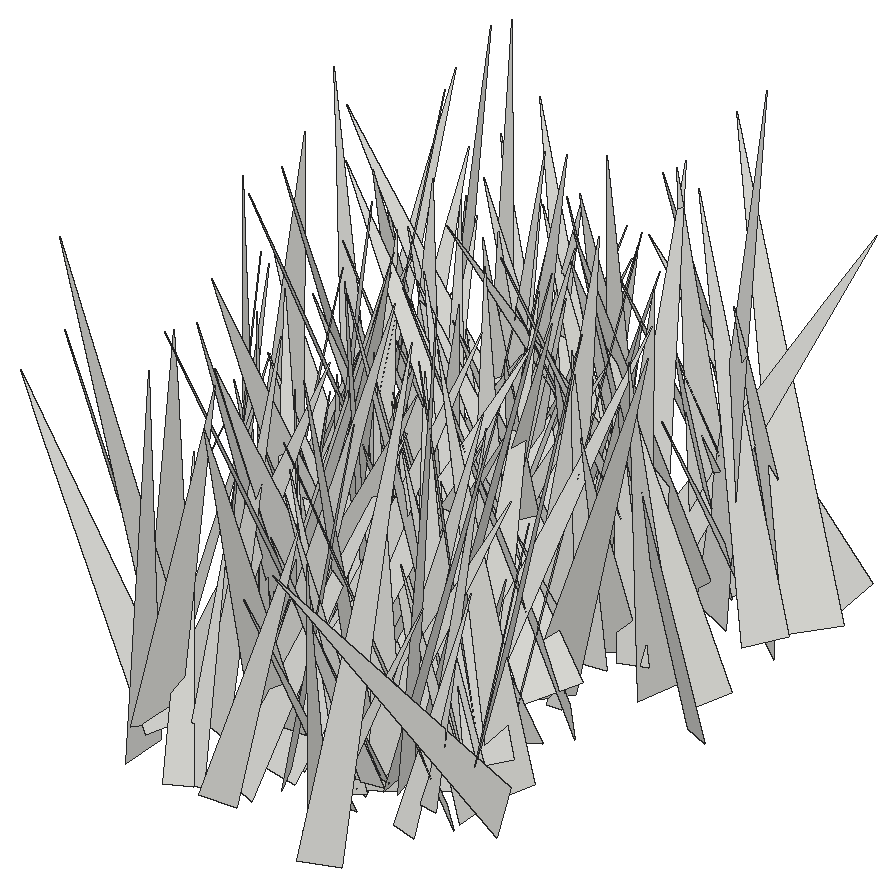
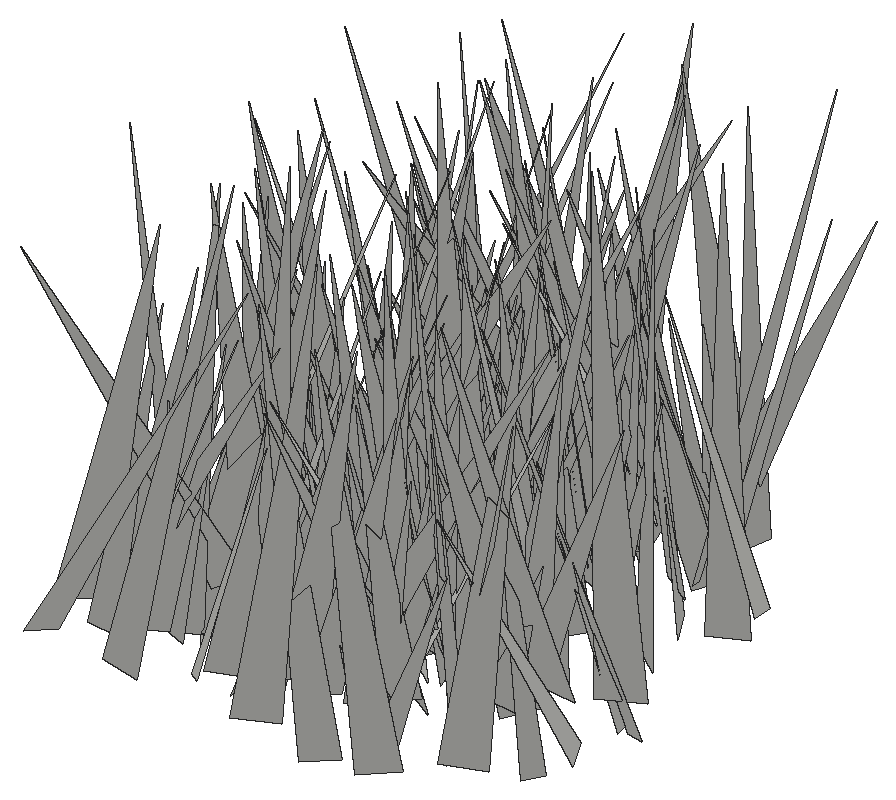
# SketchUp Ruby script. Lengths in inches.
U = 1.inch
M = Sketchup.active_model
def pt(a) = Geom::Point3d.new(a.map { |v| v * U })
def face(e, loops, mat)
  f = e.add_face(loops[0].map { |a| pt(a) })
  loops[1..].each { |l| e.add_face(l.map { |a| pt(a) }).erase! }
  f.material = f.back_material = mat if mat
  f
end
# faces: each face lists its corners as indices into pts; further lists are holes
def faces(e, pts, list, mat = nil) = list.each { |f| face(e, (f[0].is_a?(Array) ? f : [f]).map { |l| l.map { |i| pts[i] } }, mat) }
# xy, xz, yz: faces in a plane at the given z, y or x. An outline is a flat list of corners, or four numbers for a rectangle; further outlines are holes
def ring(l) = l.size == 4 ? [[l[0], l[1]], [l[2], l[1]], [l[2], l[3]], [l[0], l[3]]] : l.each_slice(2).to_a
def flat(e, list, mat, &to3) = list.each { |f| face(e, (f[0].is_a?(Array) ? f : [f]).map { |l| ring(l).map { |u, v| to3.(u, v) } }, mat) }
def xy(e, z, list, mat = nil) = flat(e, list, mat) { |x, y| [x, y, z] }
def xz(e, y, list, mat = nil) = flat(e, list, mat) { |x, z| [x, y, z] }
def yz(e, x, list, mat = nil) = flat(e, list, mat) { |y, z| [x, y, z] }
def lines(e, pts, list) = list.each { |a, b| e.add_line(pt(pts[a]), pt(pts[b])) }
# prism: a flat outline (further loops are holes) pulled along v
def prism(e, loops, v, mat = nil)
  f = face(e, loops, mat); d = Geom::Vector3d.new(v.map { |x| x * U })
  f.pushpull(f.normal.samedirection?(d) ? d.length : -d.length)
end
def box(e, o, s, mat = nil) = prism(e, [[o, [o[0] + s[0], o[1], o[2]], [o[0] + s[0], o[1] + s[1], o[2]], [o[0], o[1] + s[1], o[2]]]], [0, 0, s[2]], mat)
def at(x, y, z, deg = 0) = Geom::Transformation.translation(pt([x, y, z])) * Geom::Transformation.rotation(ORIGIN, Z_AXIS, deg.degrees)
def axes(o, x, y, z) = Geom::Transformation.new([*x, 0, *y, 0, *z, 0, *pt(o).to_a, 1])
def part(name) = M.definitions.add(name)
# library, detail: a bought-in or finely detailed component or shape, given as its bounding box
def library(name, o, s) = part(name).tap { |d| box(d.entities, o, s) }
def detail(e, o, s) = box(e.add_group.entities, o, s)
def put(e, d, t, mat = nil) = e.add_instance(d, t).tap { |i| i.material = mat if mat }
def group(e, t, mat = nil) = e.add_group.tap { |g| g.transformation = t; g.material = mat if mat }.entities
root = M.entities
c1 = part("fur_instance\#9")
p = [[0.8125,0,1.79],[0.67,-0.02,1.48],[0,-0.11,0],[0,0.11,0]]
faces(c1.entities,p,[[0,1,2,3]])
put(root,c1,axes([114.01,82.89,-27.1],[-3.48001,3.233,0.8636],[3.33945,3.27515,1.19585],[-0.21495,-1.45934,4.59703]))
put(root,c1,axes([115.01,81.97,-28.22],[-7.7657,1.30292,0.44128],[1.14319,7.51969,-2.08465],[0.76515,1.98873,7.59328]))
put(root,c1,axes([111.08,82.71,-27.1],[1.84601,-7.44066,1.73932],[-7.59322,-1.58595,1.27441],[0.85535,1.97933,7.55956]))
put(root,c1,axes([111.375,84.31,-28.22],[4.18382,1.92252,0.07247],[1.86113,-4.08842,1.01327],[-0.48737,0.89131,4.49152]))
put(root,c1,axes([113.84,75.04,-28.22],[-3.86878,-4.9807,0.99535],[-5.05831,3.89149,-0.18804],[0.45997,0.9025,6.30392]))
put(root,c1,axes([111.3125,82.24,-28.22],[4.10602,0.97464,0.35289],[0.9844,-4.11806,-0.08026],[-0.32469,-0.15985,4.21935]))
put(root,c1,axes([113.36,78.78,-28.22],[-3.98091,-5.38333,3.048],[-6.04161,4.16252,-0.53901],[1.33021,2.79489,6.67363]))
put(root,c1,axes([112.16,88.45,-27.1],[2.77965,-6.05851,0.20454],[-6.05263,-2.78627,-0.276],[-0.3362,0.0706,6.66001]))
put(root,c1,axes([114.03,86.49,-28.22],[-5.31437,-1.63311,1.48269],[-1.72892,5.48589,-0.1545],[1.36976,0.58821,5.55749]))
put(root,c1,axes([112.81,83.5,-27.1],[0.72086,7.11073,0.81641],[7.15729,-0.71063,-0.13028],[0.04812,-0.82534,7.14599]))
put(root,c1,axes([111.1,76.29,-27.1],[4.64757,1.11707,0.03174],[1.0994,-4.54603,-0.98676],[0.20042,-0.96672,4.67697]))
put(root,c1,axes([111.49,86.13,-28.22],[4.97063,-0.22915,0.23226],[-0.15729,-4.7897,-1.3593],[-0.28585,-1.34904,4.78665]))
put(root,c1,axes([110.68,82.55,-28.22],[3.86219,5.07234,0.99731],[5.04282,-3.42294,-2.11973],[1.1372,-2.04809,6.01264]))
put(root,c1,axes([114.9375,73.96,-28.22],[-7.82049,-1.65264,1.82204],[-1.48703,8.01344,0.88582],[1.95953,-0.51451,7.94397]))
put(root,c1,axes([114.15,79.39,-27.1],[-0.09942,-3.58739,1.13729],[-3.70553,-0.10534,-0.65623],[-0.65715,1.13676,3.52826]))
put(root,c1,axes([115.83,71.83,-27.1],[-4.20776,3.77593,1.0344],[3.85861,3.7428,2.0336],[-0.66241,-2.18328,5.27517]))
put(root,c1,axes([112.23,76.42,-28.22],[1.17808,-6.7396,1.1437],[-6.76699,-0.98532,1.16408],[0.96855,1.31342,6.74203]))
put(root,c1,axes([113.92,76.64,-27.1],[2.58353,5.00263,1.49189],[5.09313,-2.78069,0.50442],[-1.14546,-1.08079,5.60772]))
put(root,c1,axes([113.47,85.05,-27.1],[-3.16063,-7.46069,0.64697],[-7.21635,3.22195,1.90087],[2.00118,-0.16476,7.87643]))
put(root,c1,axes([114.02,83.35,-28.22],[-4.09876,5.0884,1.14662],[4.86258,4.25523,-1.50159],[1.8873,0.0873,6.359]))
put(root,c1,axes([113.66,76.76,-28.22],[5.69134,3.55142,2.30083],[3.82093,-5.97012,-0.23634],[-1.81848,-1.42926,6.70433]))
put(root,c1,axes([115.77,87.57,-28.22],[-1.40668,3.30295,0.84871],[3.29754,1.08331,1.24951],[-0.86952,-1.23511,3.36556]))
put(root,c1,axes([114.84,85.45,-28.22],[2.73063,4.59292,1.67983],[4.59916,-3.06583,0.90635],[-1.66266,-0.93747,5.2659]))
put(root,c1,axes([113.47,74.68,-28.22],[3.62165,4.35293,0.90177],[4.41878,-3.65214,-0.11732],[-0.48531,-0.76904,5.66132]))
put(root,c1,axes([118,86.58,-27.1],[-6.653,2.83628,0.09553],[2.75112,6.38619,1.99099],[-0.69638,-1.86767,6.95291]))
put(root,c1,axes([113.74,78.61,-28.22],[5.547,2.87669,1.51326],[2.93945,-5.71712,0.09337],[-1.38744,-0.61131,6.24786]))
put(root,c1,axes([113.97,82.125,-27.1],[6.26441,4.08516,1.86388],[4.05019,-6.52197,0.68206],[-1.9387,-0.42509,7.44756]))
put(root,c1,axes([117.06,84.14,-27.1],[-4.69197,-2.31538,0.05263],[-2.28134,4.60011,-1.00642],[-0.39908,0.92541,5.13447]))
put(root,c1,axes([113.85,86.6,-27.1],[4.80804,6.17674,2.98381],[6.78482,-4.81897,-0.95722],[-1.01068,-2.96612,7.76873]))
put(root,c1,axes([114.67,78.89,-28.22],[3.09566,2.75124,1.27433],[2.88928,-3.22895,-0.04754],[-0.91941,-0.88367,4.14127]))
put(root,c1,axes([114.35,81.55,-28.22],[-0.50328,-4.91347,1.0032],[-4.85841,0.72759,1.12622],[1.24277,0.85458,4.80907]))
put(root,c1,axes([113.6875,82.86,-27.1],[3.31192,-3.28223,0.0309],[-3.2384,-3.26025,0.79144],[0.53549,0.5836,4.59516]))
put(root,c1,axes([114.97,71.86,-28.22],[6.40054,-0.55178,2.21578],[-0.37829,-6.75939,-0.5905],[-2.25189,-0.43282,6.39709]))
put(root,c1,axes([115.65,81,-28.22],[3.27303,-4.65782,3.06275],[-5.40234,-3.52629,0.41046],[-1.37496,2.76738,5.67799]))
put(root,c1,axes([116.7,86.33,-27.1],[0.17252,3.92598,1.26935],[3.97591,-0.49782,0.99933],[-1.10305,-1.18034,3.80058]))
put(root,c1,axes([116.94,70.99,-28.22],[-0.56854,4.75375,0.07359],[4.64609,0.5398,1.02436],[-1.0087,-0.19303,4.67676]))
put(root,c1,axes([117.125,74.75,-27.1],[2.66286,4.62658,1.9724],[4.32664,-3.24515,1.77077],[-2.56433,-0.67099,5.03592]))
put(root,c1,axes([117.53,82.47,-28.22],[-0.4063,-5.76079,1.26429],[-5.69006,0.04941,-1.60344],[-1.5519,1.32705,5.54804]))
put(root,c1,axes([115.4,83.625,-27.1],[-4.12278,4.06528,3.37823],[4.64279,4.83304,-0.14992],[2.52655,-2.24755,5.78803]))
put(root,c1,axes([115.35,83.12,-27.1],[4.3108,-3.69492,0.61953],[-3.55093,-4.33068,-1.12044],[-1.19463,-0.46051,5.56597]))
put(root,c1,axes([115.95,86.48,-27.1],[-2.49427,4.27012,1.59064],[4.35584,2.76683,-0.59729],[1.33819,-1.04698,4.90903]))
put(root,c1,axes([116.23,79.43,-28.22],[-1.82022,-4.66244,0.24993],[-4.60062,1.83672,0.75812],[0.79693,-0.04591,4.9474]))
put(root,c1,axes([118.17,79.37,-28.22],[-5.398,0.07669,0.31538],[0.11355,5.36878,0.63804],[0.30406,-0.64352,5.36071]))
put(root,c1,axes([116.02,81.65,-27.1],[0.74131,3.87524,0.12897],[3.87698,-0.74271,0.03187],[-0.05555,-0.12068,3.94537]))
put(root,c1,axes([117.64,84.39,-27.1],[-7.86516,0.65945,1.92725],[0.13584,7.83978,-2.12819],[2.03241,2.02799,7.60042]))
put(root,c1,axes([116.52,79.46,-27.1],[4.04445,-6.42376,0.8146],[-6.13253,-4.10829,-1.94934],[-2.07854,-0.37835,7.33638]))
put(root,c1,axes([118.85,85.53,-27.1],[-2.09774,5.99421,0.07606],[5.73274,1.98235,1.88224],[-1.75272,-0.69034,6.06533]))
put(root,c1,axes([114.4375,74.19,-28.22],[4.48664,-4.30175,1.96808],[-4.72578,-3.95369,2.13158],[0.21294,2.89338,5.83878]))
put(root,c1,axes([119.46,80.21,-27.1],[-4.9129,-5.75828,0.52895],[-5.68371,4.68095,-1.83254],[-1.06438,1.58274,7.34412]))
put(root,c1,axes([117.32,80.84,-28.22],[-4.47188,4.60163,0.40246],[4.4512,4.44255,-1.33612],[1.23441,0.65071,6.27595]))
put(root,c1,axes([116.75,84.74,-28.22],[2.36342,5.34352,0.74133],[5.25737,-2.46286,0.99138],[-1.20944,-0.26392,5.75813]))
put(root,c1,axes([115.07,88.625,-28.22],[2.93008,-5.46925,1.49234],[-5.65269,-2.69042,1.23848],[0.43226,1.89052,6.07982]))
put(root,c1,axes([117.7,76.23,-28.22],[-2.53564,-6.45433,1.27855],[-6.57975,2.48748,-0.49186],[0.00081,1.3699,6.91708]))
put(root,c1,axes([116.08,78.94,-27.1],[0.58274,-3.68979,0.92218],[-3.78198,-0.46356,0.53511],[0.40205,0.98748,3.697]))
put(root,c1,axes([117.64,84.19,-27.1],[-4.95355,2.49117,1.9463],[2.93301,4.97148,1.10159],[1.17959,-1.90003,5.43416]))
put(root,c1,axes([117.44,82.47,-27.1],[-0.20928,5.81187,1.2771],[5.90875,0.05179,0.73257],[-0.70395,-1.2931,5.76932]))
put(root,c1,axes([117.93,87.63,-27.1],[-5.02237,2.51021,1.68016],[2.86774,4.98644,1.12241],[0.94877,-1.78398,5.50142]))
put(root,c1,axes([117.09,83.39,-27.1],[2.12896,3.50938,0.78952],[3.35263,-2.26833,1.04217],[-1.30344,-0.10245,3.97015]))
put(root,c1,axes([117.5,85.57,-28.22],[0.74185,-5.118,0.35857],[-5.01336,-0.80012,-1.04825],[-1.09027,0.19676,5.06413]))
put(root,c1,axes([118.375,74.35,-28.22],[-2.09458,6.39775,0.76013],[6.40195,1.97698,1.00139],[-0.72385,-1.02792,6.657]))
put(root,c1,axes([118.24,83.51,-27.1],[-3.93894,0.78438,0.2139],[0.7314,3.88076,-0.76228],[0.35506,0.70765,3.94328]))
put(root,c1,axes([115.47,71.77,-27.1],[5.59181,-3.37862,1.09906],[-3.46581,-5.63815,0.30113],[-0.78177,0.82912,6.52631]))
put(root,c1,axes([119.2,84.67,-27.1],[-3.24563,2.42896,0.17461],[2.25293,2.88449,1.75171],[-0.92447,-1.49811,3.65588]))
put(root,c1,axes([117.23,71.24,-28.22],[0.0321,3.78164,0.61426],[3.82721,-0.05969,0.16749],[-0.17489,-0.6122,3.77806]))
put(root,c1,axes([114.43,82.59,-27.1],[3.95823,-3.37287,0.12226],[-3.1364,-3.60629,2.0534],[1.24667,1.63622,4.7778]))
put(root,c1,axes([117.3,76.52,-27.1],[4.85297,5.01471,2.08252],[4.89411,-5.24941,1.23566],[-2.35199,-0.5761,6.86817]))
put(root,c1,axes([118.98,87.44,-27.1],[-4.49285,4.90641,0.97236],[5.00159,4.41981,0.80831],[0.04935,-1.26349,6.60342]))
put(root,c1,axes([117.89,75.23,-28.22],[2.91004,3.86675,2.0314],[3.84438,-3.42612,1.0144],[-2.0734,-0.92551,4.73192]))
put(root,c1,axes([117.26,79.01,-27.1],[-0.85461,3.70026,0.75554],[3.7566,0.91253,-0.21994],[0.38824,-0.68446,3.79129]))
put(root,c1,axes([118.72,77.03,-28.22],[-3.73085,2.02538,0.45172],[2.07172,3.68874,0.57157],[0.11914,-0.71871,4.20651]))
put(root,c1,axes([117.43,73.35,-27.1],[4.44404,5.53922,0.27989],[5.13876,-4.2472,2.46279],[-2.08674,1.3376,6.66087]))
put(root,c1,axes([116.55,86.46,-27.1],[3.89931,-1.45547,0.98195],[-1.58431,-3.9476,0.44006],[-0.75669,0.76505,4.13877]))
put(root,c1,axes([114.58,80.71,-27.1],[8.18505,-1.50624,0.16494],[-1.43272,-7.98824,-1.85106],[-0.49323,-1.79175,8.11402]))
put(root,c1,axes([116.97,72.54,-27.1],[1.78136,5.8506,1.71123],[6.09225,-1.76893,-0.29408],[-0.20572,-1.72409,6.10871]))
put(root,c1,axes([116.52,86.29,-27.1],[6.38697,-1.69717,1.73981],[-1.81592,-6.58358,0.24416],[-1.61547,0.69051,6.6041]))
put(root,c1,axes([116.13,86.17,-27.1],[4.9565,-0.0282,0.53243],[-0.1703,-4.80111,1.33099],[-0.50525,1.34155,4.77453]))
put(root,c1,axes([117.75,77.27,-27.1],[5.40513,-4.44008,1.03103],[-3.91993,-5.34397,-2.46351],[-2.32626,-1.31164,6.54682]))
put(root,c1,axes([117.26,73.52,-28.22],[-6.44163,0.17845,3.84936],[-1.24896,6.99677,-2.4144],[3.64548,2.71245,5.9747]))
put(root,c1,axes([117.03,83.07,-28.22],[5.01565,1.80166,1.23073],[1.89818,-5.12441,-0.23415],[-1.07592,-0.64182,5.32428]))
put(root,c1,axes([117.7,85.67,-28.22],[4.78165,-4.93816,1.39024],[-4.88475,-4.96331,-0.82896],[-1.56762,0.40313,6.82367]))
put(root,c1,axes([118.89,82.01,-27.1],[-6.51752,1.2418,2.00991],[0.54856,6.53189,-2.25684],[2.29801,1.9627,6.23913]))
put(root,c1,axes([117.9375,82.93,-28.22],[4.52328,4.39752,0.22155],[4.10164,-4.32376,2.0806],[-1.60118,1.34692,5.95561]))
put(root,c1,axes([119.4375,76.72,-28.22],[-1.66438,3.94539,0.96796],[4.04045,1.49913,0.83702],[-0.42169,-1.20819,4.19948]))
put(root,c1,axes([116.7,87.27,-28.22],[4.88196,1.64498,0.71636],[1.77456,-4.73338,-1.22423],[-0.26474,-1.39349,5.00407]))
put(root,c1,axes([120.58,87.08,-28.22],[-2.86629,5.19134,1.30889],[5.27356,2.48156,1.70596],[-0.92348,-1.94182,5.67938]))
put(root,c1,axes([123.125,80.125,-27.1],[-5.23637,6.32875,0.17784],[5.87309,4.76933,3.20385],[-2.36465,-2.16904,7.5636]))
put(root,c1,axes([116.79,89.1,-28.22],[1.45023,-6.39796,1.08768],[-6.25164,-1.07813,1.99368],[1.74182,1.45734,6.24998]))
put(root,c1,axes([119.58,79.47,-27.1],[-3.58724,1.8714,1.40372],[2.1412,3.66165,0.59026],[0.94225,-1.19623,4.00275]))
put(root,c1,axes([118.4,89.99,-27.1],[4.15376,-5.21591,0.7578],[-5.12927,-4.22232,-0.94677],[-1.21268,-0.00681,6.60024]))
put(root,c1,axes([122.48,73.26,-27.1],[-4.6508,-5.63712,0.37429],[-5.36466,4.25457,-2.58191],[-1.77136,1.91537,6.83673]))
put(root,c1,axes([118.26,74.14,-28.22],[2.6634,-7.09113,0.13913],[-7.08626,-2.66678,-0.26525],[-0.29724,0.03689,7.57017]))
put(root,c1,axes([119.32,76.79,-27.1],[3.99412,4.65299,3.2629],[5.30006,-4.48907,-0.08624],[-2.05092,-2.53923,6.13155]))
put(root,c1,axes([120.35,84.67,-27.1],[-0.32554,-5.06602,0.7464],[-4.99056,0.14633,-1.18345],[-1.14716,0.80105,4.9366]))
put(root,c1,axes([118.37,82.47,-27.1],[5.34451,-1.51745,2.02584],[-2.07356,-5.33917,1.4711],[-1.45157,2.03988,5.35746]))
put(root,c1,axes([118.58,76.02,-28.22],[0.82444,4.69785,1.50621],[4.90559,-0.61872,-0.75536],[0.52313,-1.60174,4.70945]))
put(root,c1,axes([119.89,89.18,-27.1],[-6.50454,-4.83681,0.42708],[-4.2184,5.98256,3.50717],[2.40464,-2.5885,7.30777]))
put(root,c1,axes([121.99,82.82,-27.1],[-4.61226,3.61546,0.79034],[3.61757,4.1381,2.18138],[-0.78062,-2.18488,5.43931]))
put(root,c1,axes([121.13,73.64,-28.22],[-0.23432,4.6061,1.3303],[4.44797,-0.2882,1.78136],[-1.78924,-1.31967,4.25416]))
put(root,c1,axes([121.64,82,-28.22],[-3.53792,4.34861,0.23075],[4.30519,3.44804,1.02808],[-0.65501,-0.82532,5.51093]))
put(root,c1,axes([116.39,76.3,-27.1],[2.55754,-6.5759,0.86107],[-6.14173,-2.00015,2.96707],[2.50263,1.81158,6.40156]))
put(root,c1,axes([119.24,81.99,-28.22],[1.49528,-4.80686,1.53266],[-5.04418,-1.45777,0.34917],[-0.10564,1.56838,5.02194]))
put(root,c1,axes([118.39,70.94,-28.22],[2.49544,-4.2024,1.5625],[-4.46283,-2.15679,1.32672],[0.42981,2.0042,4.70396]))
put(root,c1,axes([119.33,79.54,-28.22],[4.3427,-1.50818,1.19732],[-1.3579,-4.49272,-0.73402],[-1.36538,-0.32877,4.53816]))
put(root,c1,axes([118.36,71.88,-28.22],[1.55452,5.85258,0.28483],[5.77094,-1.47817,-1.12324],[1.01494,-0.55917,5.95042]))
put(root,c1,axes([117.89,74,-27.1],[2.9133,6.77269,2.26525],[7.08174,-2.424,-1.8604],[0.9217,-2.7826,7.13411]))
put(root,c1,axes([118.09,78.1,-27.1],[4.70172,-1.10111,0.26171],[-1.12934,-4.49092,1.39405],[0.07438,1.41645,4.62334]))
put(root,c1,axes([120.67,79.5,-27.1],[-3.88391,-3.01754,1.00768],[-2.99103,4.00531,0.46572],[1.08383,0.24005,4.89626]))
put(root,c1,axes([120.93,80.13,-28.22],[-4.05728,-2.523,0.42943],[-2.40041,4.03064,1.00168],[0.88766,-0.63233,4.67158]))
put(root,c1,axes([118.04,81.03,-28.22],[2.3597,-7.64104,0.82634],[-7.58316,-2.17409,1.55097],[1.25061,1.23463,7.84527]))
put(root,c1,axes([119.06,73.24,-28.22],[5.44742,2.57642,1.57153],[2.74581,-5.57692,-0.37485],[-1.25227,-1.0208,6.0143]))
put(root,c1,axes([117.92,82.8,-27.1],[2.74788,4.31889,0.7575],[4.17328,-2.30167,-2.01583],[1.34551,-1.68135,4.70533]))
put(root,c1,axes([120.26,75.51,-28.22],[-2.6676,-6.3456,1.58153],[-6.4273,2.85927,0.63121],[1.20736,1.20081,6.85451]))
put(root,c1,axes([120.92,77.4375,-27.1],[1.65267,-3.08975,1.39314],[-3.11179,-1.99748,-0.7386],[-1.34319,0.82596,3.42525]))
put(root,c1,axes([118.23,74.3,-28.22],[2.2285,7.10603,0.93052],[7.02267,-1.97084,-1.76797],[1.42959,-1.39565,7.23438]))
put(root,c1,axes([119.15,84.38,-28.22],[4.70982,-4.44224,0.12242],[-4.38661,-4.67586,-0.90827],[-0.71149,-0.57769,6.41023]))
put(root,c1,axes([121.51,72.93,-28.22],[-1.12963,-3.6746,0.26296],[-3.62855,1.06225,-0.74377],[-0.63679,0.46567,3.77168]))
put(root,c1,axes([117.98,77.38,-27.1],[4.10331,-3.61689,0.17449],[-3.47529,-3.85943,1.7253],[1.0172,1.40442,5.19061]))
put(root,c1,axes([121.07,86.98,-27.1],[-3.83453,-4.44323,0.31037],[-4.29048,3.7947,1.3169],[1.19597,-0.63261,5.71941]))
put(root,c1,axes([118.22,82.44,-28.22],[6.83641,-1.96558,0.32372],[-1.94381,-6.83529,-0.45298],[-0.43579,-0.34652,7.09893]))
put(root,c1,axes([122.11,73.01,-27.1],[-1.05055,-3.99645,1.56356],[-4.12582,0.49771,-1.49997],[-1.18067,1.81677,3.85037]))
put(root,c1,axes([120.68,80.43,-27.1],[-1.61639,5.70202,2.80279],[6.31476,1.76115,0.05886],[0.70173,-2.71416,5.92641]))
put(root,c1,axes([120.18,87.26,-27.1],[-0.4517,-7.27096,2.0225],[-7.50286,0.65147,0.6664],[0.81515,1.96726,7.25444]))
put(root,c1,axes([118.4,73.26,-28.22],[-2.61013,7.00123,1.33294],[6.01827,2.92557,-3.58165],[3.81765,0.17478,6.55758]))
put(root,c1,axes([120.26,85.3,-27.1],[0.02895,-4.95019,0.58964],[-4.94989,0.0415,0.59139],[0.59214,0.58889,4.91483]))
put(root,c1,axes([122.39,73.54,-27.1],[-5.96382,1.04535,0.88629],[0.82737,5.90096,-1.39268],[1.09259,1.23747,5.8924]))
put(root,c1,axes([121.32,89.12,-27.1],[-2.38013,-2.88459,0.25848],[-2.75196,2.35686,0.96161],[0.90246,-0.42079,3.61403]))
put(root,c1,axes([122.23,82.2,-27.1],[-4.07436,-2.22938,0.28557],[-2.14023,4.02883,0.91657],[0.68639,-0.67121,4.55307]))
put(root,c1,axes([120.68,84.79,-28.22],[1.57919,4.13225,1.33364],[4.34025,-1.54395,-0.35548],[-0.12772,-1.37428,4.40942]))
put(root,c1,axes([120.62,88.4,-27.1],[5.40488,-4.57462,0.50738],[-4.27322,-5.27816,-2.06831],[-1.71004,-1.26929,6.77215]))
put(root,c1,axes([123.73,76.07,-28.22],[-7.0839,-2.86843,1.00142],[-2.98784,7.03787,-0.97651],[0.55097,1.28563,7.57997]))
put(root,c1,axes([122.43,72.85,-27.1],[-0.63614,-4.28295,0.71253],[-4.25699,0.4736,-0.95381],[-0.85404,0.8295,4.22357]))
put(root,c1,axes([120.86,72.33,-28.22],[4.7247,0.27251,1.48983],[0.66278,-4.76043,-1.23114],[-1.36183,-1.37139,4.56961]))
put(root,c1,axes([120.86,83.55,-28.22],[3.83115,1.46002,1.29175],[1.69697,-3.89964,-0.62537],[-0.95945,-1.06731,4.05194]))
put(root,c1,axes([122.8,76.88,-28.22],[-5.92228,3.52878,0.304],[3.26745,5.67188,-2.1844],[1.36692,1.73077,6.53866]))
put(root,c1,axes([120.14,82.57,-28.22],[6.55283,1.12937,1.12544],[0.97488,-6.60494,0.95181],[-1.26162,0.76214,6.58096]))
put(root,c1,axes([123.19,79.05,-28.22],[-0.67131,-4.1889,0.93111],[-4.10147,0.34927,-1.38579],[-1.26165,1.09345,4.00962]))
put(root,c1,axes([122.39,81.1,-28.22],[2.07794,4.44656,0.23399],[4.16362,-2.03187,1.63715],[-1.57826,0.49406,4.62704]))
put(root,c1,axes([124.27,75.82,-27.1],[-6.63605,2.7216,0.19643],[2.70208,6.62626,-0.52374],[0.38006,0.41041,7.15332]))
put(root,c1,axes([123.34,80.73,-28.22],[-5.81753,-5.50464,0.89808],[-5.45533,5.88597,0.73893],[1.16061,0.07452,7.97488]))
put(root,c1,axes([122.49,85.1,-27.1],[-1.30736,-3.53096,1.01989],[-3.67333,1.2908,-0.2398],[0.12042,1.04076,3.75757]))
put(root,c1,axes([123.49,84.37,-27.1],[-4.0044,1.49429,0.5536],[1.5481,4.00291,0.3933],[0.37782,-0.56428,4.25599]))
put(root,c1,axes([122.83,75.28,-28.22],[-2.98056,5.41129,1.99239],[5.72855,3.03527,0.32601],[0.65987,-1.90801,6.16924]))
put(root,c1,axes([121.27,82.37,-27.1],[5.02607,-4.57327,2.19343],[-4.92834,-5.13329,0.59007],[-1.19892,1.92923,6.76964]))
put(root,c1,axes([123.91,85.57,-28.22],[-5.96811,-4.81477,0.42538],[-4.75156,5.96808,0.88657],[0.88638,-0.42578,7.61672]))
put(root,c1,axes([121.52,74.25,-28.22],[-4.5359,3.17744,2.60533],[2.766,5.23085,-1.56386],[3.0386,-0.01843,5.3127]))
put(root,c1,axes([124.09,74.31,-28.22],[-4.64993,-4.92524,0.42817],[-4.93518,4.6591,-0.00251],[0.29211,0.31306,6.77347]))
put(root,c1,axes([124.3,75.35,-28.22],[-0.71726,5.0627,1.58469],[5.02661,0.13746,1.836],[-1.69568,-1.73401,4.77227]))
put(root,c1,axes([120.21,85.06,-28.22],[6.88515,-2.28469,0.18682],[-2.24647,-6.84269,-0.88939],[-0.45618,-0.78602,7.19959]))
put(root,c1,axes([122.98,82,-27.1],[-0.34045,4.62028,2.07312],[5.05885,0.21591,0.34957],[-0.23002,-2.08976,4.6196]))
put(root,c1,axes([121.32,78.47,-28.22],[3.62629,-0.3933,0.08931],[-0.3696,-3.56406,-0.68808],[-0.16141,-0.67481,3.58206]))
put(root,c1,axes([122.66,84.28,-27.1],[-3.77046,5.93467,2.17976],[6.06315,4.1134,-0.71146],[1.79161,-1.43096,6.99504]))
put(root,c1,axes([122.88,86.99,-27.1],[-0.43608,-7.58063,0.50958],[-7.59761,0.43802,0.01424],[0.04352,0.50791,7.59315]))
put(root,c1,axes([120.65,74.1,-28.22],[0.50211,5.33526,1.29674],[5.04367,0.06639,-2.22613],[2.16978,-1.38897,4.87457]))
put(root,c1,axes([123.23,90.08,-27.1],[-2.01035,-7.12989,1.00319],[-7.18316,2.0575,0.22838],[0.49393,0.90254,7.40437]))
put(root,c1,axes([123.17,73.43,-27.1],[-6.34859,-2.07949,3.15929],[-2.7531,6.77324,-1.07409],[2.59343,2.09974,6.59357]))
put(root,c1,axes([123.23,87.65,-27.1],[-1.72033,-4.15588,1.09836],[-4.2769,1.77348,0.01157],[0.4311,1.01028,4.49785]))
put(root,c1,axes([125.57,87.6,-27.1],[-2.41735,-5.08882,0.8159],[-4.81582,1.90935,-2.35956],[-1.83565,1.69223,5.11586]))
put(root,c1,axes([121.87,85.02,-27.1],[3.13383,-5.16211,1.39491],[-5.34355,-3.08346,0.59403],[-0.19921,1.50298,6.00961]))
put(root,c1,axes([123.58,76.39,-28.22],[-4.72321,-4.87597,2.05821],[-5.0831,4.94763,0.05633],[1.47426,1.43735,6.78828]))
put(root,c1,axes([124.12,68.35,-27.1],[-7.01528,2.7432,0.95764],[2.14491,6.5776,-3.12905],[1.96,2.6204,6.85188]))
put(root,c1,axes([123.34,87.44,-27.1],[3.99451,-5.40043,2.70776],[-5.64329,-4.49426,-0.63847],[-2.15638,1.75774,6.68679]))
put(root,c1,axes([123.87,82.8,-27.1],[-0.78367,4.54033,1.31363],[4.69244,0.5877,0.76808],[-0.56674,-1.41222,4.54299]))
put(root,c1,axes([124.6,76.51,-28.22],[-6.49588,1.72746,1.45223],[1.82521,6.62397,0.28488],[1.32729,-0.65455,6.71561]))
put(root,c1,axes([122.9,69.54,-27.1],[-3.04551,1.64304,1.0176],[0.80196,2.80235,-2.12461],[1.7584,1.56764,2.73144]))
put(root,c1,axes([124.52,74.57,-28.22],[-3.89073,-0.42692,0.42553],[-0.44504,3.90915,-0.14719],[0.40654,0.19356,3.91132]))
put(root,c1,axes([121.8,77.87,-27.1],[1.69788,6.23349,0.03172],[6.16311,-1.67374,-0.97718],[0.93461,-0.28707,6.38626]))
put(root,c1,axes([124.52,88.74,-27.1],[-3.87512,-3.17972,0.32504],[-3.163,3.88842,0.32938],[0.4601,-0.04943,5.00187]))
put(root,c1,axes([122.5,77.5,-28.22],[3.65523,2.01923,0.98653],[2.16689,-3.66612,-0.52479],[-0.59594,-0.94526,4.14277]))
put(root,c1,axes([122.39,75.1,-27.1],[7.1658,2.76652,1.69463],[2.58302,-7.35112,1.0785],[-1.96302,0.42601,7.60521]))
put(root,c1,axes([122.86,73.2,-27.1],[5.61181,2.09612,1.30854],[1.89864,-5.73587,1.04566],[-1.58152,0.55181,5.89854]))
put(root,c1,axes([123.16,83.2,-27.1],[2.62732,-3.98087,0.28129],[-3.95197,-2.64215,-0.47983],[-0.55532,-0.03119,4.74551]))
put(root,c1,axes([123.23,77.74,-28.22],[6.37842,4.90538,1.53696],[4.59516,-6.53882,1.79932],[-2.30422,0.53885,7.84279]))
put(root,c1,axes([126.39,89.7,-27.1],[-6.42762,0.7775,0.36666],[0.8533,6.10569,2.01137],[0.10407,-2.04186,6.15412]))
put(root,c1,axes([125.62,84.11,-28.22],[-5.32926,2.77314,1.19327],[2.9808,5.21718,1.1879],[0.47858,-1.6143,5.88899]))
put(root,c1,axes([125.96,86.17,-27.1],[-6.07575,2.79462,0.62219],[2.80321,6.10345,-0.04049],[0.58225,-0.22305,6.68752]))
put(root,c1,axes([124.49,72.76,-27.1],[2.31766,5.02687,0.82298],[4.84651,-2.45447,1.34356],[-1.56781,-0.15629,5.3699]))
put(root,c1,axes([120.92,85.59,-28.22],[-0.59602,7.49567,1.64856],[6.68012,1.32078,-3.59019],[3.77872,-1.15261,6.60687]))
put(root,c1,axes([126.58,82.29,-28.22],[-5.12266,-6.1706,2.10185],[-6.50165,4.64284,-2.21548],[-0.47189,3.01719,7.70776]))
put(root,c1,axes([123.87,86.34,-27.1],[3.41828,7.22194,2.57308],[7.56489,-3.63472,0.1519],[-1.24484,-2.25703,7.98861]))
put(root,c1,axes([123.57,72.84,-28.22],[0.71871,3.7725,0.80138],[3.83913,-0.62217,-0.51422],[0.36739,-0.87844,3.80576]))
put(root,c1,axes([125.16,87.54,-28.22],[-3.4189,-2.83051,0.24342],[-2.77437,3.40847,0.66713],[0.61145,-0.36118,4.38812]))
put(root,c1,axes([123.53,76.05,-28.22],[6.24718,3.3719,1.68528],[3.2403,-6.4703,0.93425],[-1.92623,0.05148,7.03734]))
put(root,c1,axes([126.6,87.54,-27.1],[-5.45873,5.352,1.02249],[5.44819,5.38274,0.9113],[0.08123,-1.36725,7.5902]))
put(root,c1,axes([121.97,81.4,-28.22],[6.42408,-3.63909,0.41323],[-3.66082,-6.40525,0.50369],[-0.11006,0.64215,7.36601]))
put(root,c1,axes([125.1,75.45,-28.22],[-6.54697,-3.05595,0.68846],[-2.14459,5.53525,4.1758],[2.28332,-3.56338,5.89613]))
put(root,c1,axes([124.18,83.55,-28.22],[5.42089,-2.3865,1.81758],[-2.19868,-5.71457,-0.94576],[-2.04078,-0.18248,5.84696]))
put(root,c1,axes([125.02,88.58,-27.1],[-0.19276,-5.01478,1.27598],[-5.16585,0.1124,-0.33865],[-0.30027,1.28555,5.00705]))
